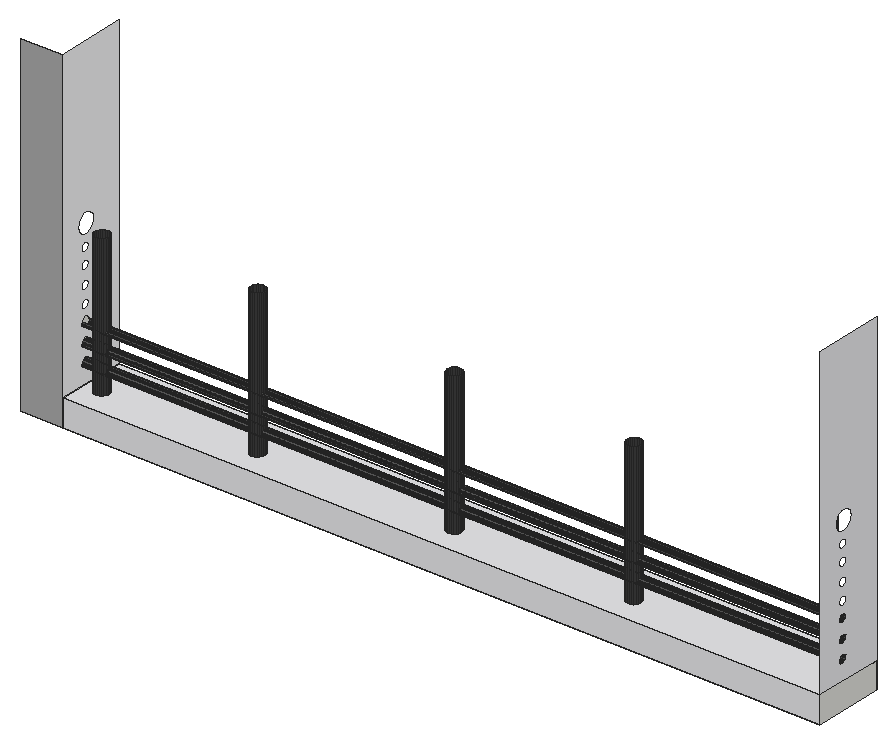
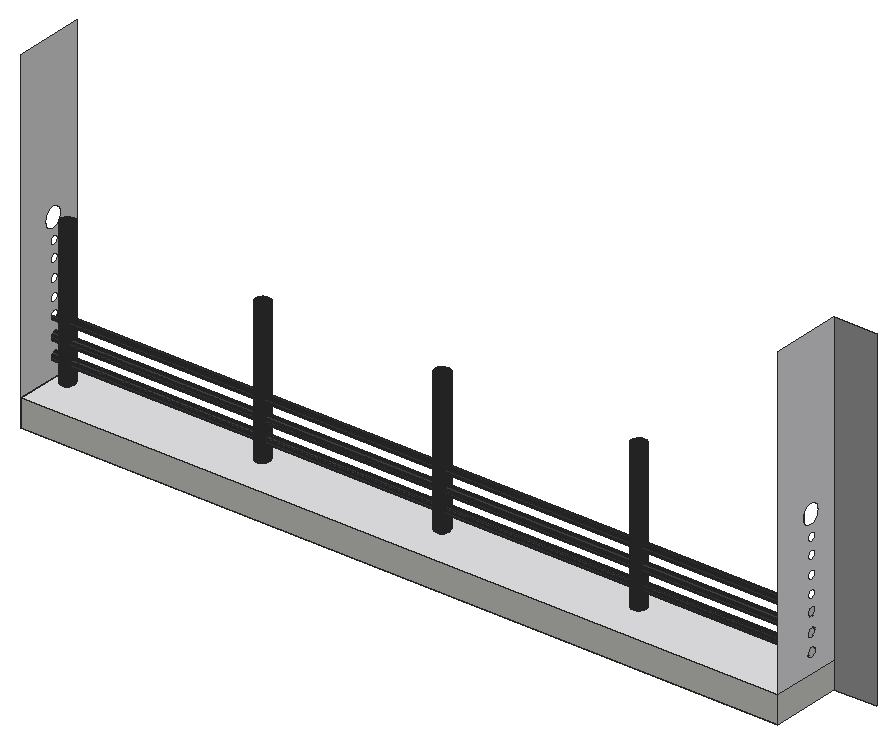
# SketchUp Ruby script. Lengths in inches.
U = 1.inch
M = Sketchup.active_model
def pt(a) = Geom::Point3d.new(a.map { |v| v * U })
def face(e, loops, mat)
  f = e.add_face(loops[0].map { |a| pt(a) })
  loops[1..].each { |l| e.add_face(l.map { |a| pt(a) }).erase! }
  f.material = f.back_material = mat if mat
  f
end
# faces: each face lists its corners as indices into pts; further lists are holes
def faces(e, pts, list, mat = nil) = list.each { |f| face(e, (f[0].is_a?(Array) ? f : [f]).map { |l| l.map { |i| pts[i] } }, mat) }
# xy, xz, yz: faces in a plane at the given z, y or x. An outline is a flat list of corners, or four numbers for a rectangle; further outlines are holes
def ring(l) = l.size == 4 ? [[l[0], l[1]], [l[2], l[1]], [l[2], l[3]], [l[0], l[3]]] : l.each_slice(2).to_a
def flat(e, list, mat, &to3) = list.each { |f| face(e, (f[0].is_a?(Array) ? f : [f]).map { |l| ring(l).map { |u, v| to3.(u, v) } }, mat) }
def xy(e, z, list, mat = nil) = flat(e, list, mat) { |x, y| [x, y, z] }
def xz(e, y, list, mat = nil) = flat(e, list, mat) { |x, z| [x, y, z] }
def yz(e, x, list, mat = nil) = flat(e, list, mat) { |y, z| [x, y, z] }
def lines(e, pts, list) = list.each { |a, b| e.add_line(pt(pts[a]), pt(pts[b])) }
# prism: a flat outline (further loops are holes) pulled along v
def prism(e, loops, v, mat = nil)
  f = face(e, loops, mat); d = Geom::Vector3d.new(v.map { |x| x * U })
  f.pushpull(f.normal.samedirection?(d) ? d.length : -d.length)
end
def box(e, o, s, mat = nil) = prism(e, [[o, [o[0] + s[0], o[1], o[2]], [o[0] + s[0], o[1] + s[1], o[2]], [o[0], o[1] + s[1], o[2]]]], [0, 0, s[2]], mat)
def at(x, y, z, deg = 0) = Geom::Transformation.translation(pt([x, y, z])) * Geom::Transformation.rotation(ORIGIN, Z_AXIS, deg.degrees)
def axes(o, x, y, z) = Geom::Transformation.new([*x, 0, *y, 0, *z, 0, *pt(o).to_a, 1])
def part(name) = M.definitions.add(name)
# library, detail: a bought-in or finely detailed component or shape, given as its bounding box
def library(name, o, s) = part(name).tap { |d| box(d.entities, o, s) }
def detail(e, o, s) = box(e.add_group.entities, o, s)
def put(e, d, t, mat = nil) = e.add_instance(d, t).tap { |i| i.material = mat if mat }
def group(e, t, mat = nil) = e.add_group.tap { |g| g.transformation = t; g.material = mat if mat }.entities
root = M.entities
M.materials.add("[Blinds Vertical Pattern]").color = [245, 245, 247]
M.materials.add("[Blinds Vertical Pattern]1").color = [232, 232, 234]
M.materials.add("[Blinds Vertical Pattern]2").color = [234, 234, 237]
M.materials.add("[Color M03]").color = [170, 170, 170]
M.materials.add("[Color M06]").color = [86, 86, 86]
M.materials.add("[Color M07]").color = [58, 58, 58]
xy(root,703.5,[[56.39,446.5625,415.32,480.02]])
xy(root,715.9375,[[64.24,456.35,63.39,456.58,62.62,457.01,62,457.63,61.55,458.39,61.32,459.24,61.31,460.125,61.54,460.98,61.98,461.74,62.6,462.37,63.36,462.8125,64.21,463.05,65.09,463.05,65.9375,462.83,66.7,462.39,67.33,461.77,67.77,461.01,68.01,460.16,68.01,459.28,67.79,458.43,67.35,457.66,66.73,457.03,65.97,456.59,65.12,456.36],[137.99,456.35,137.14,456.58,136.37,457.01,135.75,457.63,135.3,458.39,135.07,459.24,135.06,460.125,135.29,460.98,135.73,461.74,136.35,462.37,137.11,462.8125,137.96,463.05,138.84,463.05,139.6875,462.83,140.45,462.39,141.08,461.77,141.52,461.01,141.76,460.16,141.76,459.28,141.54,458.43,141.1,457.66,140.48,457.03,139.72,456.59,138.87,456.36],[231.18,456.35,230.32,456.58,229.56,457.01,228.93,457.63,228.49,458.39,228.26,459.24,228.25,460.125,228.48,460.98,228.91,461.74,229.53,462.37,230.29,462.8125,231.14,463.05,232.02,463.05,232.875,462.83,233.64,462.39,234.27,461.77,234.71,461.01,234.94,460.16,234.95,459.28,234.73,458.43,234.29,457.66,233.67,457.03,232.91,456.59,232.06,456.36],[316.36,456.35,315.51,456.58,314.75,457.01,314.12,457.63,313.68,458.39,313.44,459.24,313.44,460.125,313.66,460.98,314.1,461.74,314.72,462.37,315.48,462.8125,316.33,463.05,317.21,463.05,318.0625,462.83,318.83,462.39,319.46,461.77,319.9,461.01,320.13,460.16,320.14,459.28,319.91,458.43,319.48,457.66,318.86,457.03,318.1,456.59,317.25,456.36],[408.8,456.35,407.95,456.58,407.18,457.01,406.56,457.63,406.11,458.39,405.88,459.24,405.88,460.125,406.1,460.98,406.54,461.74,407.16,462.37,407.92,462.8125,408.77,463.05,409.65,463.05,410.5,462.83,411.27,462.39,411.89,461.77,412.34,461.01,412.57,460.16,412.57,459.28,412.35,458.43,411.91,457.66,411.29,457.03,410.53,456.59,409.68,456.36]])
xy(root,715.9375,[[[56.39,446.5625,415.32,480.02],[64.24,456.35,63.39,456.58,62.62,457.01,62,457.63,61.55,458.39,61.32,459.24,61.31,460.125,61.54,460.98,61.98,461.74,62.6,462.37,63.36,462.8125,64.21,463.05,65.09,463.05,65.9375,462.83,66.7,462.39,67.33,461.77,67.77,461.01,68.01,460.16,68.01,459.28,67.79,458.43,67.35,457.66,66.73,457.03,65.97,456.59,65.12,456.36],[408.8,456.35,407.95,456.58,407.18,457.01,406.56,457.63,406.11,458.39,405.88,459.24,405.88,460.125,406.1,460.98,406.54,461.74,407.16,462.37,407.92,462.8125,408.77,463.05,409.65,463.05,410.5,462.83,411.27,462.39,411.89,461.77,412.34,461.01,412.57,460.16,412.57,459.28,412.35,458.43,411.91,457.66,411.29,457.03,410.53,456.59,409.68,456.36],[137.99,456.35,137.14,456.58,136.37,457.01,135.75,457.63,135.3,458.39,135.07,459.24,135.06,460.125,135.29,460.98,135.73,461.74,136.35,462.37,137.11,462.8125,137.96,463.05,138.84,463.05,139.6875,462.83,140.45,462.39,141.08,461.77,141.52,461.01,141.76,460.16,141.76,459.28,141.54,458.43,141.1,457.66,140.48,457.03,139.72,456.59,138.87,456.36],[316.36,456.35,315.51,456.58,314.75,457.01,314.12,457.63,313.68,458.39,313.44,459.24,313.44,460.125,313.66,460.98,314.1,461.74,314.72,462.37,315.48,462.8125,316.33,463.05,317.21,463.05,318.0625,462.83,318.83,462.39,319.46,461.77,319.9,461.01,320.13,460.16,320.14,459.28,319.91,458.43,319.48,457.66,318.86,457.03,318.1,456.59,317.25,456.36],[231.18,456.35,230.32,456.58,229.56,457.01,228.93,457.63,228.49,458.39,228.26,459.24,228.25,460.125,228.48,460.98,228.91,461.74,229.53,462.37,230.29,462.8125,231.14,463.05,232.02,463.05,232.875,462.83,233.64,462.39,234.27,461.77,234.71,461.01,234.94,460.16,234.95,459.28,234.73,458.43,234.29,457.66,233.67,457.03,232.91,456.59,232.06,456.36]]],"[Blinds Vertical Pattern]1")
xz(root,446.5625,[[56.39,703.5,415.32,715.9375]],"[Blinds Vertical Pattern]1")
xz(root,446.5625,[[36.42,703.5,56.39,861.625]],"[Color M03]")
xz(root,463.05,[[64.21,715.9375,65.09,782.625],[137.96,715.9375,138.84,785.43],[231.14,715.9375,232.02,782.97],[316.33,715.9375,317.21,782.97],[408.77,715.9375,409.65,784.2]],"[Color M07]")
xz(root,480.02,[[56.39,703.5,415.32,715.9375]])
yz(root,56.39,[[446.5625,703.5,480.02,715.9375],[459.98,723.35,459.46,723.42,458.98,723.62,458.57,723.93,458.25,724.35,458.05,724.83,457.98,725.35,458.05,725.87,458.25,726.35,458.57,726.76,458.98,727.08,459.46,727.28,459.98,727.35,460.5,727.28,460.98,727.08,461.39,726.76,461.71,726.35,461.91,725.87,461.98,725.35,461.91,724.83,461.71,724.35,461.39,723.93,460.98,723.62,460.5,723.42],[459.98,731.79,459.46,731.85,458.98,732.05,458.57,732.37,458.25,732.79,458.05,733.27,457.98,733.79,458.05,734.3,458.25,734.79,458.57,735.2,458.98,735.52,459.46,735.72,459.98,735.79,460.5,735.72,460.98,735.52,461.39,735.2,461.71,734.79,461.91,734.3,461.98,733.79,461.91,733.27,461.71,732.79,461.39,732.37,460.98,732.05,460.5,731.85],[459.98,740.66,459.46,740.73,458.98,740.93,458.57,741.25,458.25,741.66,458.05,742.14,457.98,742.66,458.05,743.18,458.25,743.66,458.57,744.07,458.98,744.39,459.46,744.59,459.98,744.66,460.5,744.59,460.98,744.39,461.39,744.07,461.71,743.66,461.91,743.18,461.98,742.66,461.91,742.14,461.71,741.66,461.39,741.25,460.98,740.93,460.5,740.73]])
yz(root,56.39,[[[446.5625,715.9375,480.02,861.625],[460.55,779.45,459.32,779.61,458.18,780.09,457.2,780.84,456.44,781.83,455.97,782.97,455.8,784.2,455.97,785.43,456.44,786.58,457.2,787.56,458.18,788.31,459.32,788.79,460.55,788.95,461.78,788.79,462.93,788.31,463.91,787.56,464.67,786.58,465.14,785.43,465.3,784.2,465.14,782.97,464.67,781.83,463.91,780.84,462.93,780.09,461.78,779.61],[459.98,723.35,459.46,723.42,458.98,723.62,458.57,723.93,458.25,724.35,458.05,724.83,457.98,725.35,458.05,725.87,458.25,726.35,458.57,726.76,458.98,727.08,459.46,727.28,459.98,727.35,460.5,727.28,460.98,727.08,461.39,726.76,461.71,726.35,461.91,725.87,461.98,725.35,461.91,724.83,461.71,724.35,461.39,723.93,460.98,723.62,460.5,723.42],[459.98,772.35,459.46,772.42,458.98,772.62,458.57,772.93,458.25,773.35,458.05,773.83,457.98,774.35,458.05,774.87,458.25,775.35,458.57,775.76,458.98,776.08,459.46,776.28,459.98,776.35,460.5,776.28,460.98,776.08,461.39,775.76,461.71,775.35,461.91,774.87,461.98,774.35,461.91,773.83,461.71,773.35,461.39,772.93,460.98,772.62,460.5,772.42],[459.98,731.79,459.46,731.85,458.98,732.05,458.57,732.37,458.25,732.79,458.05,733.27,457.98,733.79,458.05,734.3,458.25,734.79,458.57,735.2,458.98,735.52,459.46,735.72,459.98,735.79,460.5,735.72,460.98,735.52,461.39,735.2,461.71,734.79,461.91,734.3,461.98,733.79,461.91,733.27,461.71,732.79,461.39,732.37,460.98,732.05,460.5,731.85],[459.98,764.6,459.46,764.67,458.98,764.87,458.57,765.18,458.25,765.6,458.05,766.08,457.98,766.6,458.05,767.12,458.25,767.6,458.57,768.01,458.98,768.33,459.46,768.53,459.98,768.6,460.5,768.53,460.98,768.33,461.39,768.01,461.71,767.6,461.91,767.12,461.98,766.6,461.91,766.08,461.71,765.6,461.39,765.18,460.98,764.87,460.5,764.67],[459.98,740.66,459.46,740.73,458.98,740.93,458.57,741.25,458.25,741.66,458.05,742.14,457.98,742.66,458.05,743.18,458.25,743.66,458.57,744.07,458.98,744.39,459.46,744.59,459.98,744.66,460.5,744.59,460.98,744.39,461.39,744.07,461.71,743.66,461.91,743.18,461.98,742.66,461.91,742.14,461.71,741.66,461.39,741.25,460.98,740.93,460.5,740.73],[459.98,756.16,459.46,756.23,458.98,756.43,458.57,756.75,458.25,757.16,458.05,757.64,457.98,758.16,458.05,758.68,458.25,759.16,458.57,759.57,458.98,759.89,459.46,760.09,459.98,760.16,460.5,760.09,460.98,759.89,461.39,759.57,461.71,759.16,461.91,758.68,461.98,758.16,461.91,757.64,461.71,757.16,461.39,756.75,460.98,756.43,460.5,756.23],[459.98,747.97,459.46,748.04,458.98,748.24,458.57,748.56,458.25,748.97,458.05,749.46,457.98,749.97,458.05,750.49,458.25,750.97,458.57,751.39,458.98,751.71,459.46,751.9,459.98,751.97,460.5,751.9,460.98,751.71,461.39,751.39,461.71,750.97,461.91,750.49,461.98,749.97,461.91,749.46,461.71,748.97,461.39,748.56,460.98,748.24,460.5,748.04]]],"[Blinds Vertical Pattern]")
yz(root,68.01,[[459.28,715.9375,460.16,782.625]],"[Color M07]")
yz(root,141.76,[[459.28,715.9375,460.16,785.43]],"[Color M07]")
yz(root,313.44,[[459.24,715.9375,460.125,782.97]],"[Color M07]")
yz(root,405.88,[[459.24,715.9375,460.125,784.2]],"[Color M07]")
yz(root,412.57,[[459.28,715.9375,460.16,784.2]],"[Color M07]")
yz(root,415.32,[[446.5625,703.5,480.02,715.9375]])
yz(root,415.32,[[[446.5625,715.9375,480.02,861.625],[460.55,779.45,461.78,779.61,462.93,780.09,463.91,780.84,464.67,781.83,465.14,782.97,465.3,784.2,465.14,785.43,464.67,786.58,463.91,787.56,462.93,788.31,461.78,788.79,460.55,788.95,459.32,788.79,458.18,788.31,457.2,787.56,456.44,786.58,455.97,785.43,455.8,784.2,455.97,782.97,456.44,781.83,457.2,780.84,458.18,780.09,459.32,779.61],[459.98,723.35,460.5,723.42,460.98,723.62,461.39,723.93,461.71,724.35,461.91,724.83,461.98,725.35,461.91,725.87,461.71,726.35,461.39,726.76,460.98,727.08,460.5,727.28,459.98,727.35,459.46,727.28,458.98,727.08,458.57,726.76,458.25,726.35,458.05,725.87,457.98,725.35,458.05,724.83,458.25,724.35,458.57,723.93,458.98,723.62,459.46,723.42],[459.98,731.79,460.5,731.85,460.98,732.05,461.39,732.37,461.71,732.79,461.91,733.27,461.98,733.79,461.91,734.3,461.71,734.79,461.39,735.2,460.98,735.52,460.5,735.72,459.98,735.79,459.46,735.72,458.98,735.52,458.57,735.2,458.25,734.79,458.05,734.3,457.98,733.79,458.05,733.27,458.25,732.79,458.57,732.37,458.98,732.05,459.46,731.85],[459.98,740.66,460.5,740.73,460.98,740.93,461.39,741.25,461.71,741.66,461.91,742.14,461.98,742.66,461.91,743.18,461.71,743.66,461.39,744.07,460.98,744.39,460.5,744.59,459.98,744.66,459.46,744.59,458.98,744.39,458.57,744.07,458.25,743.66,458.05,743.18,457.98,742.66,458.05,742.14,458.25,741.66,458.57,741.25,458.98,740.93,459.46,740.73],[459.98,747.97,460.5,748.04,460.98,748.24,461.39,748.56,461.71,748.97,461.91,749.46,461.98,749.97,461.91,750.49,461.71,750.97,461.39,751.39,460.98,751.71,460.5,751.9,459.98,751.97,459.46,751.9,458.98,751.71,458.57,751.39,458.25,750.97,458.05,750.49,457.98,749.97,458.05,749.46,458.25,748.97,458.57,748.56,458.98,748.24,459.46,748.04],[459.98,756.16,460.5,756.23,460.98,756.43,461.39,756.75,461.71,757.16,461.91,757.64,461.98,758.16,461.91,758.68,461.71,759.16,461.39,759.57,460.98,759.89,460.5,760.09,459.98,760.16,459.46,760.09,458.98,759.89,458.57,759.57,458.25,759.16,458.05,758.68,457.98,758.16,458.05,757.64,458.25,757.16,458.57,756.75,458.98,756.43,459.46,756.23],[459.98,764.6,460.5,764.67,460.98,764.87,461.39,765.18,461.71,765.6,461.91,766.08,461.98,766.6,461.91,767.12,461.71,767.6,461.39,768.01,460.98,768.33,460.5,768.53,459.98,768.6,459.46,768.53,458.98,768.33,458.57,768.01,458.25,767.6,458.05,767.12,457.98,766.6,458.05,766.08,458.25,765.6,458.57,765.18,458.98,764.87,459.46,764.67],[459.98,772.35,460.5,772.42,460.98,772.62,461.39,772.93,461.71,773.35,461.91,773.83,461.98,774.35,461.91,774.87,461.71,775.35,461.39,775.76,460.98,776.08,460.5,776.28,459.98,776.35,459.46,776.28,458.98,776.08,458.57,775.76,458.25,775.35,458.05,774.87,457.98,774.35,458.05,773.83,458.25,773.35,458.57,772.93,458.98,772.62,459.46,772.42]]],"[Blinds Vertical Pattern]2")
p = [[63.39,456.58,715.9375],[64.24,456.35,715.9375],[64.24,456.35,782.625],[63.39,456.58,782.625],[65.12,456.36,715.9375],[65.12,456.36,782.625],
  [65.97,456.59,715.9375],[65.97,456.59,782.625],[137.14,456.58,715.9375],[137.99,456.35,715.9375],[137.99,456.35,785.43],[137.14,456.58,785.43],
  [138.87,456.36,715.9375],[138.87,456.36,785.43],[139.72,456.59,715.9375],[139.72,456.59,785.43],[230.32,456.58,715.9375],[231.18,456.35,715.9375],
  [231.18,456.35,782.97],[230.32,456.58,782.97],[232.06,456.36,715.9375],[232.06,456.36,782.97],[232.91,456.59,715.9375],[232.91,456.59,782.97],
  [315.51,456.58,715.9375],[316.36,456.35,715.9375],[316.36,456.35,782.97],[315.51,456.58,782.97],[317.25,456.36,715.9375],[317.25,456.36,782.97],
  [318.1,456.59,715.9375],[318.1,456.59,782.97],[407.95,456.58,715.9375],[408.8,456.35,715.9375],[408.8,456.35,784.2],[407.95,456.58,784.2],
  [409.68,456.36,715.9375],[409.68,456.36,784.2],[410.53,456.59,715.9375],[410.53,456.59,784.2],[62.62,457.01,715.9375],[62.62,457.01,782.625],
  [66.73,457.03,715.9375],[66.73,457.03,782.625],[136.37,457.01,715.9375],[136.37,457.01,785.43],[140.48,457.03,715.9375],[140.48,457.03,785.43],
  [229.56,457.01,715.9375],[229.56,457.01,782.97],[233.67,457.03,715.9375],[233.67,457.03,782.97],[314.75,457.01,715.9375],[314.75,457.01,782.97],
  [318.86,457.03,715.9375],[318.86,457.03,782.97],[407.18,457.01,715.9375],[407.18,457.01,784.2],[411.29,457.03,715.9375],[411.29,457.03,784.2],
  [62,457.63,715.9375],[62,457.63,782.625],[67.35,457.66,715.9375],[67.35,457.66,782.625],[135.75,457.63,715.9375],[135.75,457.63,785.43],
  [141.1,457.66,715.9375],[141.1,457.66,785.43],[228.93,457.63,715.9375],[228.93,457.63,782.97],[234.29,457.66,715.9375],[234.29,457.66,782.97],
  [314.12,457.63,715.9375],[314.12,457.63,782.97],[319.48,457.66,715.9375],[319.48,457.66,782.97],[406.56,457.63,715.9375],[406.56,457.63,784.2],
  [411.91,457.66,715.9375],[411.91,457.66,784.2],[61.55,458.39,715.9375],[61.55,458.39,782.625],[135.3,458.39,715.9375],[135.3,458.39,785.43],
  [228.49,458.39,715.9375],[228.49,458.39,782.97],[313.68,458.39,715.9375],[313.68,458.39,782.97],[406.11,458.39,715.9375],[406.11,458.39,784.2],
  [67.79,458.43,715.9375],[67.79,458.43,782.625],[141.54,458.43,715.9375],[141.54,458.43,785.43],[234.73,458.43,715.9375],[234.73,458.43,782.97],
  [319.91,458.43,715.9375],[319.91,458.43,782.97],[412.35,458.43,715.9375],[412.35,458.43,784.2],[61.32,459.24,715.9375],[61.32,459.24,782.625],
  [68.01,459.28,715.9375],[68.01,459.28,782.625],[135.07,459.24,715.9375],[135.07,459.24,785.43],[141.76,459.28,715.9375],[141.76,459.28,785.43],
  [228.26,459.24,715.9375],[228.26,459.24,782.97],[234.95,459.28,715.9375],[234.95,459.28,782.97],[313.44,459.24,715.9375],[313.44,459.24,782.97],
  [320.14,459.28,715.9375],[320.14,459.28,782.97],[405.88,459.24,715.9375],[405.88,459.24,784.2],[412.57,459.28,715.9375],[412.57,459.28,784.2],
  [61.31,460.125,715.9375],[61.31,460.125,782.625],[135.06,460.125,715.9375],[135.06,460.125,785.43],[228.25,460.125,715.9375],[228.25,460.125,782.97],
  [234.94,460.16,715.9375],[234.94,460.16,782.97],[320.13,460.16,715.9375],[320.13,460.16,782.97],[61.54,460.98,715.9375],[61.54,460.98,782.625],
  [135.29,460.98,715.9375],[135.29,460.98,785.43],[228.48,460.98,715.9375],[228.48,460.98,782.97],[313.66,460.98,715.9375],[313.44,460.125,715.9375],
  [313.44,460.125,782.97],[313.66,460.98,782.97],[406.1,460.98,715.9375],[405.88,460.125,715.9375],[405.88,460.125,784.2],[406.1,460.98,784.2],
  [68.01,460.16,715.9375],[67.77,461.01,715.9375],[67.77,461.01,782.625],[68.01,460.16,782.625],[141.76,460.16,715.9375],[141.52,461.01,715.9375],
  [141.52,461.01,785.43],[141.76,460.16,785.43],[234.71,461.01,715.9375],[234.71,461.01,782.97],[319.9,461.01,715.9375],[319.9,461.01,782.97],
  [412.57,460.16,715.9375],[412.34,461.01,715.9375],[412.34,461.01,784.2],[412.57,460.16,784.2],[61.98,461.74,715.9375],[61.98,461.74,782.625],
  [67.33,461.77,715.9375],[67.33,461.77,782.625],[135.73,461.74,715.9375],[135.73,461.74,785.43],[141.08,461.77,715.9375],[141.08,461.77,785.43],
  [228.91,461.74,715.9375],[228.91,461.74,782.97],[234.27,461.77,715.9375],[234.27,461.77,782.97],[314.1,461.74,715.9375],[314.1,461.74,782.97],
  [319.46,461.77,715.9375],[319.46,461.77,782.97],[406.54,461.74,715.9375],[406.54,461.74,784.2],[411.89,461.77,715.9375],[411.89,461.77,784.2],
  [62.6,462.37,715.9375],[62.6,462.37,782.625],[136.35,462.37,715.9375],[136.35,462.37,785.43],[229.53,462.37,715.9375],[229.53,462.37,782.97],
  [314.72,462.37,715.9375],[314.72,462.37,782.97],[407.16,462.37,715.9375],[407.16,462.37,784.2],[66.7,462.39,715.9375],[66.7,462.39,782.625],
  [140.45,462.39,715.9375],[140.45,462.39,785.43],[233.64,462.39,715.9375],[233.64,462.39,782.97],[318.83,462.39,715.9375],[318.83,462.39,782.97],
  [411.27,462.39,715.9375],[411.27,462.39,784.2],[63.36,462.8125,715.9375],[63.36,462.8125,782.625],[65.9375,462.83,715.9375],[65.9375,462.83,782.625],
  [137.11,462.8125,715.9375],[137.11,462.8125,785.43],[139.6875,462.83,715.9375],[139.6875,462.83,785.43],[230.29,462.8125,715.9375],[230.29,462.8125,782.97],
  [232.875,462.83,715.9375],[232.875,462.83,782.97],[315.48,462.8125,715.9375],[315.48,462.8125,782.97],[318.0625,462.83,715.9375],[318.0625,462.83,782.97],
  [407.92,462.8125,715.9375],[407.92,462.8125,784.2],[410.5,462.83,715.9375],[410.5,462.83,784.2],[64.21,463.05,715.9375],[64.21,463.05,782.625],
  [65.09,463.05,715.9375],[65.09,463.05,782.625],[137.96,463.05,715.9375],[137.96,463.05,785.43],[138.84,463.05,715.9375],[138.84,463.05,785.43],
  [231.14,463.05,715.9375],[231.14,463.05,782.97],[232.02,463.05,715.9375],[232.02,463.05,782.97],[316.33,463.05,715.9375],[316.33,463.05,782.97],
  [317.21,463.05,715.9375],[317.21,463.05,782.97],[408.77,463.05,715.9375],[408.77,463.05,784.2],[409.65,463.05,715.9375],[409.65,463.05,784.2],
  [56.39,459.46,723.42],[56.39,459.98,723.35],[415.32,459.98,723.35],[415.32,459.46,723.42],[56.39,460.5,723.42],[415.32,460.5,723.42],
  [56.39,458.98,723.62],[415.32,458.98,723.62],[56.39,460.98,723.62],[415.32,460.98,723.62],[56.39,458.57,723.93],[415.32,458.57,723.93],
  [56.39,461.39,723.93],[415.32,461.39,723.93],[56.39,458.25,724.35],[415.32,458.25,724.35],[56.39,461.71,724.35],[415.32,461.71,724.35],
  [56.39,458.05,724.83],[415.32,458.05,724.83],[56.39,461.91,724.83],[415.32,461.91,724.83],[56.39,457.98,725.35],[415.32,457.98,725.35],
  [56.39,461.98,725.35],[415.32,461.98,725.35],[56.39,458.05,725.87],[415.32,458.05,725.87],[56.39,461.91,725.87],[415.32,461.91,725.87],
  [56.39,458.25,726.35],[415.32,458.25,726.35],[56.39,461.71,726.35],[415.32,461.71,726.35],[56.39,458.57,726.76],[415.32,458.57,726.76],
  [56.39,461.39,726.76],[415.32,461.39,726.76],[56.39,458.98,727.08],[415.32,458.98,727.08],[56.39,460.98,727.08],[415.32,460.98,727.08],
  [56.39,459.46,727.28],[415.32,459.46,727.28],[56.39,460.5,727.28],[415.32,460.5,727.28],[56.39,459.98,727.35],[415.32,459.98,727.35],
  [56.39,459.46,731.85],[56.39,459.98,731.79],[415.32,459.98,731.79],[415.32,459.46,731.85],[56.39,460.5,731.85],[415.32,460.5,731.85],
  [56.39,458.98,732.05],[415.32,458.98,732.05],[56.39,460.98,732.05],[415.32,460.98,732.05],[56.39,458.57,732.37],[415.32,458.57,732.37],
  [56.39,461.39,732.37],[415.32,461.39,732.37],[56.39,458.25,732.79],[415.32,458.25,732.79],[56.39,461.71,732.79],[415.32,461.71,732.79],
  [56.39,458.05,733.27],[415.32,458.05,733.27],[56.39,461.91,733.27],[415.32,461.91,733.27],[56.39,457.98,733.79],[415.32,457.98,733.79],
  [56.39,461.98,733.79],[415.32,461.98,733.79],[56.39,458.05,734.3],[415.32,458.05,734.3],[56.39,461.91,734.3],[415.32,461.91,734.3],
  [56.39,458.25,734.79],[415.32,458.25,734.79],[56.39,461.71,734.79],[415.32,461.71,734.79],[56.39,458.57,735.2],[415.32,458.57,735.2],
  [56.39,461.39,735.2],[415.32,461.39,735.2],[56.39,458.98,735.52],[415.32,458.98,735.52],[56.39,460.98,735.52],[415.32,460.98,735.52],
  [56.39,459.46,735.72],[415.32,459.46,735.72],[56.39,460.5,735.72],[415.32,460.5,735.72],[56.39,459.98,735.79],[415.32,459.98,735.79],
  [56.39,458.98,740.93],[56.39,459.46,740.73],[415.32,459.46,740.73],[415.32,458.98,740.93],[56.39,459.98,740.66],[415.32,459.98,740.66],
  [56.39,460.5,740.73],[415.32,460.5,740.73],[56.39,460.98,740.93],[415.32,460.98,740.93],[56.39,458.57,741.25],[415.32,458.57,741.25],
  [56.39,461.39,741.25],[415.32,461.39,741.25],[56.39,458.25,741.66],[415.32,458.25,741.66],[56.39,461.71,741.66],[415.32,461.71,741.66],
  [56.39,458.05,742.14],[415.32,458.05,742.14],[56.39,461.91,742.14],[415.32,461.91,742.14],[56.39,457.98,742.66],[415.32,457.98,742.66],
  [56.39,461.98,742.66],[415.32,461.98,742.66],[56.39,458.05,743.18],[415.32,458.05,743.18],[56.39,461.91,743.18],[415.32,461.91,743.18]]
faces(root,p,[[0,1,2,3],[1,4,5,2],[4,6,7,5],[8,9,10,11],[9,12,13,10],[12,14,15,13],[16,17,18,19],[17,20,21,18],
  [20,22,23,21],[24,25,26,27],[25,28,29,26],[28,30,31,29],[32,33,34,35],[33,36,37,34],[36,38,39,37],[40,0,3,41],
  [6,42,43,7],[44,8,11,45],[14,46,47,15],[48,16,19,49],[22,50,51,23],[52,24,27,53],[30,54,55,31],[56,32,35,57],
  [38,58,59,39],[60,40,41,61],[42,62,63,43],[64,44,45,65],[46,66,67,47],[68,48,49,69],[50,70,71,51],[72,52,53,73],
  [54,74,75,55],[76,56,57,77],[58,78,79,59],[80,60,61,81],[82,64,65,83],[84,68,69,85],[86,72,73,87],[88,76,77,89],
  [62,90,91,63],[66,92,93,67],[70,94,95,71],[74,96,97,75],[78,98,99,79],[100,80,81,101],[90,102,103,91],[104,82,83,105],
  [92,106,107,93],[108,84,85,109],[94,110,111,95],[112,86,87,113],[96,114,115,97],[116,88,89,117],[98,118,119,99],[120,100,101,121],
  [122,104,105,123],[124,108,109,125],[110,126,127,111],[114,128,129,115],[130,120,121,131],[132,122,123,133],[134,124,125,135],[136,137,138,139],
  [140,141,142,143],[144,145,146,147],[148,149,150,151],[126,152,153,127],[128,154,155,129],[156,157,158,159],[160,130,131,161],[145,162,163,146],
  [164,132,133,165],[149,166,167,150],[168,134,135,169],[152,170,171,153],[172,136,139,173],[154,174,175,155],[176,140,143,177],[157,178,179,158],
  [180,160,161,181],[182,164,165,183],[184,168,169,185],[186,172,173,187],[188,176,177,189],[162,190,191,163],[166,192,193,167],[170,194,195,171],
  [174,196,197,175],[178,198,199,179],[200,180,181,201],[190,202,203,191],[204,182,183,205],[192,206,207,193],[208,184,185,209],[194,210,211,195],
  [212,186,187,213],[196,214,215,197],[216,188,189,217],[198,218,219,199],[220,200,201,221],[202,222,223,203],[224,204,205,225],[206,226,227,207],
  [228,208,209,229],[210,230,231,211],[232,212,213,233],[214,234,235,215],[236,216,217,237],[218,238,239,219]],"[Color M07]")
faces(root,p,[[240,241,242,243],[241,244,245,242],[246,240,243,247],[244,248,249,245],[250,246,247,251],[248,252,253,249],[254,250,251,255],[252,256,257,253],
  [258,254,255,259],[256,260,261,257],[262,258,259,263],[260,264,265,261],[266,262,263,267],[264,268,269,265],[270,266,267,271],[268,272,273,269],
  [274,270,271,275],[272,276,277,273],[278,274,275,279],[276,280,281,277],[282,278,279,283],[280,284,285,281],[286,282,283,287],[284,286,287,285],
  [288,289,290,291],[289,292,293,290],[294,288,291,295],[292,296,297,293],[298,294,295,299],[296,300,301,297],[302,298,299,303],[300,304,305,301],
  [306,302,303,307],[304,308,309,305],[310,306,307,311],[308,312,313,309],[314,310,311,315],[312,316,317,313],[318,314,315,319],[316,320,321,317],
  [322,318,319,323],[320,324,325,321],[326,322,323,327],[324,328,329,325],[330,326,327,331],[328,332,333,329],[334,330,331,335],[332,334,335,333],
  [336,337,338,339],[337,340,341,338],[340,342,343,341],[342,344,345,343],[346,336,339,347],[344,348,349,345],[350,346,347,351],[348,352,353,349],
  [354,350,351,355],[352,356,357,353],[358,354,355,359],[356,360,361,357],[362,358,359,363],[360,364,365,361]],"[Color M06]")
